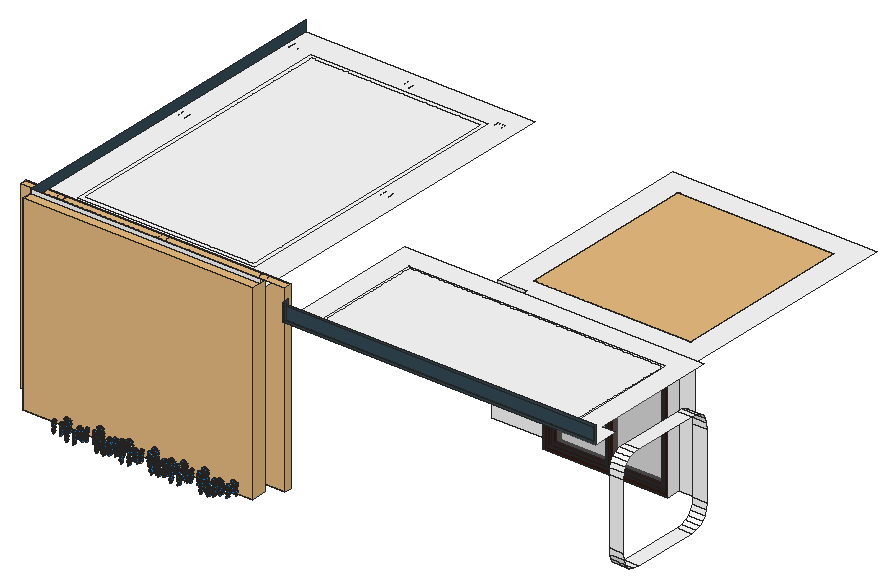
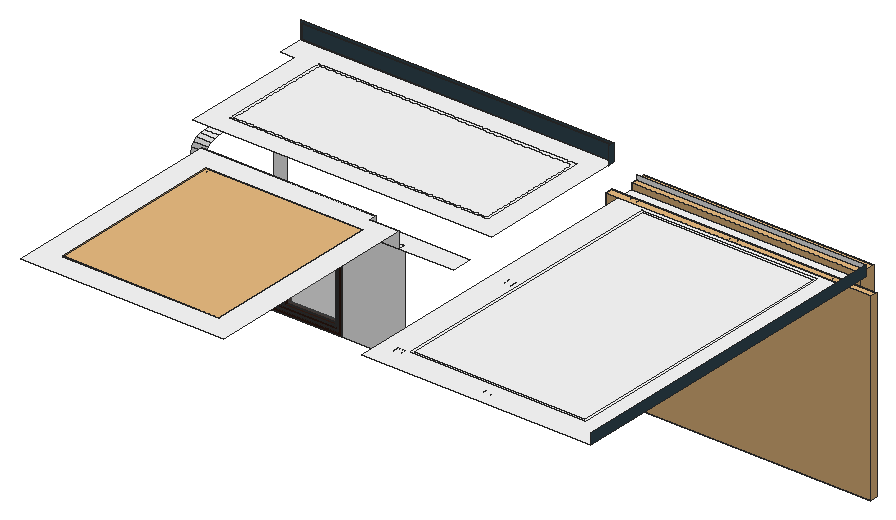
# SketchUp Ruby script. Lengths in inches.
U = 1.inch
M = Sketchup.active_model
def pt(a) = Geom::Point3d.new(a.map { |v| v * U })
def face(e, loops, mat)
  f = e.add_face(loops[0].map { |a| pt(a) })
  loops[1..].each { |l| e.add_face(l.map { |a| pt(a) }).erase! }
  f.material = f.back_material = mat if mat
  f
end
# faces: each face lists its corners as indices into pts; further lists are holes
def faces(e, pts, list, mat = nil) = list.each { |f| face(e, (f[0].is_a?(Array) ? f : [f]).map { |l| l.map { |i| pts[i] } }, mat) }
# xy, xz, yz: faces in a plane at the given z, y or x. An outline is a flat list of corners, or four numbers for a rectangle; further outlines are holes
def ring(l) = l.size == 4 ? [[l[0], l[1]], [l[2], l[1]], [l[2], l[3]], [l[0], l[3]]] : l.each_slice(2).to_a
def flat(e, list, mat, &to3) = list.each { |f| face(e, (f[0].is_a?(Array) ? f : [f]).map { |l| ring(l).map { |u, v| to3.(u, v) } }, mat) }
def xy(e, z, list, mat = nil) = flat(e, list, mat) { |x, y| [x, y, z] }
def xz(e, y, list, mat = nil) = flat(e, list, mat) { |x, z| [x, y, z] }
def yz(e, x, list, mat = nil) = flat(e, list, mat) { |y, z| [x, y, z] }
def lines(e, pts, list) = list.each { |a, b| e.add_line(pt(pts[a]), pt(pts[b])) }
# prism: a flat outline (further loops are holes) pulled along v
def prism(e, loops, v, mat = nil)
  f = face(e, loops, mat); d = Geom::Vector3d.new(v.map { |x| x * U })
  f.pushpull(f.normal.samedirection?(d) ? d.length : -d.length)
end
def box(e, o, s, mat = nil) = prism(e, [[o, [o[0] + s[0], o[1], o[2]], [o[0] + s[0], o[1] + s[1], o[2]], [o[0], o[1] + s[1], o[2]]]], [0, 0, s[2]], mat)
def at(x, y, z, deg = 0) = Geom::Transformation.translation(pt([x, y, z])) * Geom::Transformation.rotation(ORIGIN, Z_AXIS, deg.degrees)
def axes(o, x, y, z) = Geom::Transformation.new([*x, 0, *y, 0, *z, 0, *pt(o).to_a, 1])
def part(name) = M.definitions.add(name)
# library, detail: a bought-in or finely detailed component or shape, given as its bounding box
def library(name, o, s) = part(name).tap { |d| box(d.entities, o, s) }
def detail(e, o, s) = box(e.add_group.entities, o, s)
def put(e, d, t, mat = nil) = e.add_instance(d, t).tap { |i| i.material = mat if mat }
def group(e, t, mat = nil) = e.add_group.tap { |g| g.transformation = t; g.material = mat if mat }.entities
root = M.entities
M.materials.add("0496 AP 9691 Shadow-N").color = [53, 75, 86]
M.materials.add("[Color M00]").color = [255, 255, 255]
M.materials.add("[Translucent Glass Gray]").color = [128, 128, 128]
M.materials["[Translucent Glass Gray]"].alpha = 0.5
M.materials.add("lz-doorbrown").color = [51, 28, 20]
M.materials.add("skp avat flo 1").color = [0, 129, 229]
M.materials.add("skp avat flo 2").color = [47, 120, 22]
c1 = part("Gruppe\#2")
xy(c1.entities,0,[[6.69,0,4.96,0.23,3.03,1.59,1.96,1.96,0.9,3.35,0.9,5.71,0,6.69,0.23,8.43,1.96,10,3.35,12.49,4.67,13.04,7.04,12.49,8.72,13.04,10.04,12.49,11.43,11.43,12.05,9.15,13.39,6.69,13.16,4.96,12.49,3.35,10.41,2.22,8.43,0.23]],"skp avat flo 1")
c2 = part("Gruppe\#12")
xy(c2.entities,0,[[1.18,0.5,1.36,0.52,1.52,0.59,1.67,0.7,1.77,0.84,1.84,1,1.87,1.18,1.84,1.36,1.77,1.52,1.67,1.67,1.52,1.77,1.36,1.84,1.18,1.87,1,1.84,0.84,1.77,0.7,1.67,0.59,1.52,0.52,1.36,0.5,1.18,0.52,1,0.59,0.84,0.7,0.7,0.84,0.59,1,0.52]])
c3 = part("f.st. wop plant 01 blüte")
put(c3.entities,c1,at(0,0,0))
put(c3.entities,c2,at(5.65,5.41,0.39))
c4 = part("Gruppe\#5")
xy(c4.entities,0.96,[[13.97,0.22,8.73,4.42,7.37,10.11,8.43,14.53,13.97,16.39]],"skp avat flo 2")
p = [[13.97,0.22,0.96],[13.97,16.39,0.96],[17.89,14.53,4.875],[18.64,10.11,5.625],[17.67,4.42,4.66]]
faces(c4.entities,p,[[0,1,2,3,4]],"skp avat flo 2")
c5 = part("f.st. wop plant 01 blatt")
put(c5.entities,c4,axes([0.99,0,4.74],[0.91566,0,-0.40195],[0,1,0],[0.40195,0,0.91566]))
c6 = part("Gruppe\#10")
put(c6.entities,c3,axes([4.61,0.45,57.14],[0.99373,-0.06775,-0.08889],[0.11172,0.62588,0.77188],[0.00335,-0.77697,0.62953]))
put(c6.entities,c3,axes([12.4,0.4,0.59],[0.70061,0.70799,-0.08889],[-0.40079,0.49353,0.77188],[0.59035,-0.50516,0.62953]))
put(c6.entities,c3,axes([24.4375,6.09,17.58],[-0.05734,0.99439,-0.08889],[-0.63495,0.03239,0.77188],[0.77043,0.1007,0.62953]))
put(c6.entities,c3,axes([1.11,8.09,13.25],[0.88983,-0.44754,-0.08889],[0.34553,0.53368,0.77188],[-0.298,-0.71756,0.62953]))
put(c6.entities,c3,axes([23.26,15,37.53],[-0.84836,0.52191,-0.08889],[-0.38985,-0.50222,0.77188],[0.35821,0.68948,0.62953]))
put(c6.entities,c3,axes([12.67,23.61,24.88],[-0.75852,-0.64555,-0.08889],[0.35717,-0.52596,0.77188],[-0.54504,0.55374,0.62953]))
put(c6.entities,c3,axes([20.43,22.9,81.42],[-0.98432,0.15238,-0.08889],[-0.16477,-0.61405,0.77188],[0.06303,0.77442,0.62953]))
put(c6.entities,c3,axes([1.76,2.9,29.21],[0.93833,-0.33412,-0.08889],[0.27691,0.5723,0.77188],[-0.20703,-0.74889,0.62953]))
put(c6.entities,c3,axes([13.59,0.5,77.09],[0.62412,0.77625,-0.08889],[-0.4494,0.44972,0.77188],[0.63915,-0.4418,0.62953]))
put(c6.entities,c3,axes([-1.26,15.51,69.79],[0.24265,-0.96603,-0.08889],[0.62977,0.08716,0.77188],[-0.73791,-0.24328,0.62953]))
put(c6.entities,c3,axes([22.04,17.92,65.46],[-0.95793,0.27287,-0.08889],[-0.2394,-0.58898,0.77188],[0.15827,0.76069,0.62953]))
put(c6.entities,c3,axes([9.51,23.35,52.81],[-0.55554,-0.82673,-0.08889],[0.48617,-0.40969,0.77188],[-0.67455,0.38559,0.62953]))
put(c6.entities,c3,axes([0.1875,18.97,41.86],[-0.02781,-0.99565,-0.08889],[0.62986,-0.08651,0.77188],[-0.77621,-0.03452,0.62953]))
put(c6.entities,c3,axes([24.98,7.4,94.08],[-0.15925,0.98323,-0.08889],[-0.63491,-0.03305,0.77188],[0.75599,0.17936,0.62953]))
put(c6.entities,c3,axes([21.5,21.98,4.93],[-0.96344,0.25275,-0.08889],[-0.22702,-0.59386,0.77188],[0.1423,0.76384,0.62953]))
put(c6.entities,c3,axes([1.57,6.98,89.75],[0.93112,-0.3537,-0.08889],[0.28884,0.56637,0.77188],[-0.22267,-0.74439,0.62953]))
put(c6.entities,c5,axes([9.37,32.32,90.95],[-0.51317,-0.65235,0],[0.5996,-0.47167,0.32697],[-0.25699,0.20216,0.76288]))
put(c6.entities,c5,axes([33.81,6.72,78.35],[-0.27992,0.78137,0],[-0.71819,-0.25729,0.32697],[0.30782,0.11027,0.76288]))
put(c6.entities,c5,axes([-9.46,14.86,61.47],[0.53029,-0.63851,0],[0.58688,0.4874,0.32697],[-0.25154,-0.2089,0.76288]))
put(c6.entities,c5,axes([21.49,-6.15,66.98],[0.2591,0.78852,0],[-0.72476,0.23815,0.32697],[0.31063,-0.10207,0.76288]))
put(c6.entities,c5,axes([32.03,5.27,54.38],[-0.36397,0.74594,0],[-0.68562,-0.33454,0.32697],[0.29386,0.14338,0.76288]))
put(c6.entities,c5,axes([30.63,20.6,49.31],[-0.77544,0.29596,0],[-0.27203,-0.71273,0.32697],[0.11659,0.30548,0.76288]))
put(c6.entities,c5,axes([32.03,5.27,27.16],[-0.36397,0.74594,0],[-0.68562,-0.33454,0.32697],[0.29386,0.14338,0.76288]))
put(c6.entities,c5,axes([17.4375,27.53,13.8125],[-0.76735,-0.23527,0.21148],[0.29408,-0.735,0.24937],[0.11659,0.30548,0.76288]))
put(c6.entities,c5,axes([-9.46,14.86,34.24],[0.53029,-0.63851,0],[0.58688,0.4874,0.32697],[-0.25154,-0.2089,0.76288]))
c7 = part("Gruppe\#9")
put(c7.entities,c3,axes([2.2,1.62,57.61],[0.97169,-0.0623,-0.22792],[0.22172,0.57378,0.78843],[0.08166,-0.81664,0.57134]))
put(c7.entities,c3,axes([-1.48,7.53,1.27],[0.68093,0.71536,-0.15682],[-0.22028,0.40428,0.88771],[0.69843,-0.56993,0.43287]))
put(c7.entities,c3,axes([13.97,11.34,15.86],[-0.0542,0.99797,0.03349],[-0.45869,-0.05467,0.88691],[0.88694,0.03271,0.46072]))
put(c7.entities,c3,axes([-9.71,13.74,16.77],[0.84218,-0.4326,-0.32186],[0.5102,0.4462,0.73526],[-0.17446,-0.78343,0.59649]))
put(c7.entities,c3,axes([17.17,17.99,36.46],[-0.83727,0.52624,0.14846],[-0.23006,-0.58536,0.77745],[0.49603,0.61679,0.61117]))
put(c7.entities,c3,axes([4.35,27.92,27.32],[-0.77345,-0.63385,0.00301],[0.4998,-0.60694,0.61792],[-0.38984,0.47943,0.78623]))
put(c7.entities,c3,axes([20.43,22.9,81.42],[-0.98432,0.15238,-0.08889],[-0.16477,-0.61405,0.77188],[0.06303,0.77442,0.62953]))
put(c7.entities,c3,axes([-5.84,6.82,31.58],[0.89192,-0.31974,-0.31975],[0.44391,0.4844,0.75386],[-0.08616,-0.81432,0.57398]))
put(c7.entities,c3,axes([13.59,0.5,77.09],[0.62412,0.77625,-0.08889],[-0.4494,0.44972,0.77188],[0.63915,-0.4418,0.62953]))
put(c7.entities,c3,axes([-1.26,15.51,69.79],[0.24265,-0.96603,-0.08889],[0.62977,0.08716,0.77188],[-0.73791,-0.24328,0.62953]))
put(c7.entities,c3,axes([20.77,18.5,64.59],[-0.95848,0.27864,0.06062],[-0.13765,-0.63827,0.75741],[0.24973,0.71762,0.65012]))
put(c7.entities,c3,axes([6.6875,24.75,54.15],[-0.57029,-0.8188,-0.06577],[0.58283,-0.45976,0.67002],[-0.57885,0.34377,0.73942]))
put(c7.entities,c3,axes([-4.08,21.11,44.3125],[-0.04911,-0.98765,-0.14878],[0.72825,-0.13735,0.67141],[-0.68355,-0.07538,0.726]))
put(c7.entities,c3,axes([24.98,7.4,94.08],[-0.15925,0.98323,-0.08889],[-0.63491,-0.03305,0.77188],[0.75599,0.17936,0.62953]))
put(c7.entities,c3,axes([8.77,28.52,5.9],[-0.95532,0.25842,0.14346],[-0.07274,-0.676,0.7333],[0.28648,0.6901,0.6646]))
put(c7.entities,c3,axes([1.57,6.98,89.75],[0.93112,-0.3537,-0.08889],[0.28884,0.56637,0.77188],[-0.22267,-0.74439,0.62953]))
put(c7.entities,c5,axes([9.37,32.32,90.95],[-0.51317,-0.65235,0],[0.5996,-0.47167,0.32697],[-0.25699,0.20216,0.76288]))
put(c7.entities,c5,axes([33.81,6.72,78.35],[-0.27992,0.78137,0],[-0.71819,-0.25729,0.32697],[0.30782,0.11027,0.76288]))
put(c7.entities,c5,axes([-11.01,15.72,64.74],[0.51926,-0.63742,-0.11388],[0.63054,0.46456,0.27478],[-0.14729,-0.25842,0.77487]))
put(c7.entities,c5,axes([20.21,-5.625,64.6],[0.26417,0.78668,0.01588],[-0.67119,0.21655,0.43762],[0.41063,-0.15212,0.70508]))
put(c7.entities,c5,axes([29.04,6.59,51.45],[-0.35348,0.74452,0.09816],[-0.63785,-0.35493,0.39506],[0.39635,0.09281,0.72332]))
put(c7.entities,c5,axes([27.11,22.23,47.625],[-0.76537,0.29574,0.12508],[-0.23173,-0.73252,0.31403],[0.22228,0.25465,0.75805]))
put(c7.entities,c5,axes([23.375,9.49,23.48],[-0.34051,0.7404,0.15735],[-0.60881,-0.37042,0.42548],[0.44978,0.05914,0.69506]))
put(c7.entities,c5,axes([6.77,33.04,15.99],[-0.71083,-0.25923,0.3412],[0.32455,-0.75723,0.10082],[0.2798,0.21977,0.74988]))
put(c7.entities,c5,axes([-15.51,18.125,40.12],[0.50532,-0.63318,-0.18065],[0.65217,0.44994,0.24724],[-0.09068,-0.29247,0.77145]))
c8 = part("Gruppe\#11")
put(c8.entities,c3,axes([4.61,0.45,57.14],[0.99373,-0.06775,-0.08889],[0.11172,0.62588,0.77188],[0.00335,-0.77697,0.62953]))
put(c8.entities,c3,axes([12.4,0.4,0.59],[0.70061,0.70799,-0.08889],[-0.40079,0.49353,0.77188],[0.59035,-0.50516,0.62953]))
put(c8.entities,c3,axes([24.4375,6.09,17.58],[-0.05734,0.99439,-0.08889],[-0.63495,0.03239,0.77188],[0.77043,0.1007,0.62953]))
put(c8.entities,c3,axes([1.11,8.09,13.25],[0.88983,-0.44754,-0.08889],[0.34553,0.53368,0.77188],[-0.298,-0.71756,0.62953]))
put(c8.entities,c3,axes([23.26,15,37.53],[-0.84836,0.52191,-0.08889],[-0.38985,-0.50222,0.77188],[0.35821,0.68948,0.62953]))
put(c8.entities,c3,axes([12.67,23.61,24.88],[-0.75852,-0.64555,-0.08889],[0.35717,-0.52596,0.77188],[-0.54504,0.55374,0.62953]))
put(c8.entities,c3,axes([20.43,22.9,81.42],[-0.98432,0.15238,-0.08889],[-0.16477,-0.61405,0.77188],[0.06303,0.77442,0.62953]))
put(c8.entities,c3,axes([1.76,2.9,29.21],[0.93833,-0.33412,-0.08889],[0.27691,0.5723,0.77188],[-0.20703,-0.74889,0.62953]))
put(c8.entities,c3,axes([13.59,0.5,77.09],[0.62412,0.77625,-0.08889],[-0.4494,0.44972,0.77188],[0.63915,-0.4418,0.62953]))
put(c8.entities,c3,axes([-1.26,15.51,69.79],[0.24265,-0.96603,-0.08889],[0.62977,0.08716,0.77188],[-0.73791,-0.24328,0.62953]))
put(c8.entities,c3,axes([22.04,17.92,65.46],[-0.95793,0.27287,-0.08889],[-0.2394,-0.58898,0.77188],[0.15827,0.76069,0.62953]))
put(c8.entities,c3,axes([9.51,23.35,52.81],[-0.55554,-0.82673,-0.08889],[0.48617,-0.40969,0.77188],[-0.67455,0.38559,0.62953]))
put(c8.entities,c3,axes([0.1875,18.97,41.86],[-0.02781,-0.99565,-0.08889],[0.62986,-0.08651,0.77188],[-0.77621,-0.03452,0.62953]))
put(c8.entities,c3,axes([24.98,7.4,94.08],[-0.15925,0.98323,-0.08889],[-0.63491,-0.03305,0.77188],[0.75599,0.17936,0.62953]))
put(c8.entities,c3,axes([21.5,21.98,4.93],[-0.96344,0.25275,-0.08889],[-0.22702,-0.59386,0.77188],[0.1423,0.76384,0.62953]))
put(c8.entities,c3,axes([1.57,6.98,89.75],[0.93112,-0.3537,-0.08889],[0.28884,0.56637,0.77188],[-0.22267,-0.74439,0.62953]))
put(c8.entities,c5,axes([9.37,32.32,90.95],[-0.51317,-0.65235,0],[0.5996,-0.47167,0.32697],[-0.25699,0.20216,0.76288]))
put(c8.entities,c5,axes([33.81,6.72,78.35],[-0.27992,0.78137,0],[-0.71819,-0.25729,0.32697],[0.30782,0.11027,0.76288]))
put(c8.entities,c5,axes([-9.46,14.86,61.47],[0.53029,-0.63851,0],[0.58688,0.4874,0.32697],[-0.25154,-0.2089,0.76288]))
put(c8.entities,c5,axes([21.49,-6.15,66.98],[0.2591,0.78852,0],[-0.72476,0.23815,0.32697],[0.31063,-0.10207,0.76288]))
put(c8.entities,c5,axes([32.03,5.27,54.38],[-0.36397,0.74594,0],[-0.68562,-0.33454,0.32697],[0.29386,0.14338,0.76288]))
put(c8.entities,c5,axes([30.63,20.6,49.31],[-0.77544,0.29596,0],[-0.27203,-0.71273,0.32697],[0.11659,0.30548,0.76288]))
put(c8.entities,c5,axes([32.03,5.27,27.16],[-0.36397,0.74594,0],[-0.68562,-0.33454,0.32697],[0.29386,0.14338,0.76288]))
put(c8.entities,c5,axes([17.4375,27.53,13.8125],[-0.76735,-0.23527,0.21148],[0.29408,-0.735,0.24937],[0.11659,0.30548,0.76288]))
put(c8.entities,c5,axes([-9.46,14.86,34.24],[0.53029,-0.63851,0],[0.58688,0.4874,0.32697],[-0.25154,-0.2089,0.76288]))
c9 = part("Gruppe\#8")
put(c9.entities,c3,axes([2.26,1.13,59.39],[0.92531,-0.05375,-0.37538],[0.3384,0.56379,0.75341],[0.17114,-0.82417,0.53987]))
put(c9.entities,c3,axes([-9.39,6.25,4.33],[0.64151,0.72107,-0.26176],[-0.09814,0.41557,0.90425],[0.76081,-0.5544,0.33735]))
put(c9.entities,c3,axes([7.9,10.48,16.53],[-0.06325,0.99763,0.02691],[-0.32763,-0.04623,0.94367],[0.94269,0.05087,0.32978]))
put(c9.entities,c3,axes([-15.4375,12.6,20.76],[0.79424,-0.42729,-0.43198],[0.60271,0.46401,0.64918],[-0.07695,-0.77596,0.62607]))
put(c9.entities,c3,axes([13.9,17.49,36.37],[-0.81529,0.51823,0.25834],[-0.1092,-0.57574,0.81031],[0.56867,0.63242,0.52599]))
put(c9.entities,c3,axes([-0.23,27.12,29.01],[-0.75604,-0.64315,0.1215],[0.59094,-0.59091,0.5492],[-0.28142,0.48702,0.82681]))
put(c9.entities,c3,axes([20.43,22.9,81.42],[-0.98432,0.15238,-0.08889],[-0.16477,-0.61405,0.77188],[0.06303,0.77442,0.62953]))
put(c9.entities,c3,axes([-9.41,5.97,34.96],[0.84215,-0.31382,-0.43852],[0.53918,0.50168,0.67646],[0.00771,-0.80612,0.5917]))
put(c9.entities,c3,axes([13.59,0.5,77.09],[0.62412,0.77625,-0.08889],[-0.4494,0.44972,0.77188],[0.63915,-0.4418,0.62953]))
put(c9.entities,c3,axes([-1.26,15.51,69.79],[0.24265,-0.96603,-0.08889],[0.62977,0.08716,0.77188],[-0.73791,-0.24328,0.62953]))
put(c9.entities,c3,axes([22.04,17.92,65.46],[-0.95793,0.27287,-0.08889],[-0.2394,-0.58898,0.77188],[0.15827,0.76069,0.62953]))
put(c9.entities,c3,axes([6.08,24.33,55.62],[-0.57097,-0.82091,0.01051],[0.68037,-0.46598,0.56565],[-0.45945,0.33012,0.82458]))
put(c9.entities,c3,axes([-6.06,20.77,47.51],[-0.06819,-0.9857,-0.15407],[0.82323,-0.14283,0.54945],[-0.56361,-0.08937,0.8212]))
put(c9.entities,c3,axes([24.98,7.4,94.08],[-0.15925,0.98323,-0.08889],[-0.63491,-0.03305,0.77188],[0.75599,0.17936,0.62953]))
put(c9.entities,c3,axes([1.11,27.4375,7.17],[-0.92899,0.24893,0.27387],[0.04156,-0.66514,0.74556],[0.36776,0.70401,0.60756]))
put(c9.entities,c3,axes([1.57,6.98,89.75],[0.93112,-0.3537,-0.08889],[0.28884,0.56637,0.77188],[-0.22267,-0.74439,0.62953]))
put(c9.entities,c5,axes([9.37,32.32,90.95],[-0.51317,-0.65235,0],[0.5996,-0.47167,0.32697],[-0.25699,0.20216,0.76288]))
put(c9.entities,c5,axes([33.81,6.72,78.35],[-0.27992,0.78137,0],[-0.71819,-0.25729,0.32697],[0.30782,0.11027,0.76288]))
put(c9.entities,c5,axes([-9.74,15.05,68.68],[0.49765,-0.63289,-0.20172],[0.66377,0.46408,0.1815],[-0.02561,-0.27014,0.78439]))
put(c9.entities,c5,axes([21.49,-6.15,66.98],[0.2591,0.78852,0],[-0.72476,0.23815,0.32697],[0.31063,-0.10207,0.76288]))
put(c9.entities,c5,axes([27.8125,6.34,49.26],[-0.33661,0.74111,0.1623],[-0.5684,-0.36396,0.48306],[0.5025,0.08476,0.65514]))
put(c9.entities,c5,axes([25.26,22.01,46],[-0.73801,0.28975,0.24554],[-0.17833,-0.73814,0.33502],[0.33532,0.24514,0.71859]))
put(c9.entities,c5,axes([18.32,8.86,22.77],[-0.32541,0.73857,0.19371],[-0.53703,-0.37106,0.51265],[0.54278,0.07565,0.62335]))
put(c9.entities,c5,axes([0.49,32.09,17.38],[-0.65154,-0.26248,0.44214],[0.34641,-0.75151,0.06433],[0.37999,0.23503,0.69948]))
put(c9.entities,c5,axes([-17.94,17.29,44.63],[0.48369,-0.62973,-0.24163],[0.67408,0.46176,0.14595],[0.0237,-0.2813,0.78052]))
c10 = part("f.st. wop plant 01")
put(c10.entities,c6,at(39.14,64.09,18.66,-141.2))
put(c10.entities,c7,axes([53.54,120.93,12.24],[-0.61849,0.75929,0.20233],[-0.78178,-0.62056,-0.06099],[0.07925,-0.1959,0.97742]))
put(c10.entities,c8,at(82.26,36.89,18.66))
put(c10.entities,c9,axes([72.55,-5.87,29.3],[0.62579,-0.70508,0.33355],[0.76326,0.64164,-0.07566],[-0.16067,0.30193,0.93969]))
c11 = part("World of Pandora - tree 01")
put(c11.entities,c10,at(57.06,8.63,0))
c12 = library("Sliding windows",[335.6875,-0.89,0.35],[144.14,8.85,122.84])
c13 = library("шторы раздвинутые\#1",[23.6875,-79.1875,2.97],[68.3125,79.67,3.21])
c14 = part("window full")
xy(c14.entities,0,[[0,0,14.17,66.54]],"lz-doorbrown")
xy(c14.entities,2.26,[[12.2,2.26,14.17,64.28]],"lz-doorbrown")
xy(c14.entities,2.36,[[0,2.36,1.97,64.17]],"lz-doorbrown")
xy(c14.entities,3.74,[[11.42,3.74,12.2,32.875],[11.42,33.66,12.2,62.79]],"lz-doorbrown")
xy(c14.entities,3.9375,[[1.97,3.9375,2.76,32.77],[1.97,33.76,2.76,62.6]],"lz-doorbrown")
xy(c14.entities,4.18,[[2.76,4.18,7.09,32.09],[7.09,4.18,11.42,32.09],[2.76,34.45,7.09,62.35],[7.09,34.45,11.42,62.35]],"lz-doorbrown")
xy(c14.entities,69.83,[[2.76,4.18,7.09,32.09],[7.09,4.18,11.42,32.09],[7.09,32.09,11.42,34.45],[2.76,34.45,7.09,62.35],[7.09,34.45,11.42,62.35]],"lz-doorbrown")
xy(c14.entities,70.08,[[1.97,3.9375,2.76,32.77],[1.97,33.76,2.76,62.6]],"lz-doorbrown")
xy(c14.entities,70.27,[[11.42,3.74,12.2,32.875],[11.42,32.875,12.2,33.66],[11.42,33.66,12.2,62.79]],"lz-doorbrown")
xy(c14.entities,71.65,[[0,2.36,1.97,64.17]],"lz-doorbrown")
xy(c14.entities,71.76,[[12.2,2.26,14.17,64.28]],"lz-doorbrown")
xy(c14.entities,74.02,[[0,0,14.17,66.54]],"lz-doorbrown")
xz(c14.entities,0,[[0,0,14.17,74.02]],"lz-doorbrown")
xz(c14.entities,2.26,[[12.2,2.26,14.17,71.76]],"lz-doorbrown")
xz(c14.entities,2.36,[[0,2.36,1.97,71.65]],"lz-doorbrown")
xz(c14.entities,3.74,[[11.42,3.74,12.2,70.27]],"lz-doorbrown")
xz(c14.entities,3.9375,[[1.97,3.9375,2.76,70.08]],"lz-doorbrown")
xz(c14.entities,4.18,[[2.76,4.18,7.09,69.83],[7.09,4.18,11.42,69.83]],"lz-doorbrown")
xz(c14.entities,32.09,[[2.76,4.18,11.42,69.83]],"lz-doorbrown")
xz(c14.entities,32.77,[[1.97,3.9375,2.76,70.08]],"lz-doorbrown")
xz(c14.entities,32.875,[[11.42,3.74,12.2,70.27]],"lz-doorbrown")
xz(c14.entities,33.66,[[11.42,3.74,12.2,47.88],[11.42,47.88,12.2,70.27]],"lz-doorbrown")
xz(c14.entities,33.76,[[1.97,3.9375,2.76,70.08]],"lz-doorbrown")
xz(c14.entities,34.45,[[2.76,4.18,11.42,69.83]],"lz-doorbrown")
xz(c14.entities,62.35,[[2.76,4.18,7.09,69.83],[7.09,4.18,11.42,69.83]],"lz-doorbrown")
xz(c14.entities,62.6,[[1.97,3.9375,2.76,70.08]],"lz-doorbrown")
xz(c14.entities,62.79,[[11.42,3.74,12.2,70.27]],"lz-doorbrown")
xz(c14.entities,64.17,[[0,2.36,1.97,71.65]],"lz-doorbrown")
xz(c14.entities,64.28,[[12.2,2.26,14.17,71.76]],"lz-doorbrown")
xz(c14.entities,66.54,[[0,0,14.17,74.02]],"lz-doorbrown")
yz(c14.entities,0,[[[0,0,66.54,74.02],[2.36,2.36,64.17,71.65]]],"lz-doorbrown")
yz(c14.entities,1.97,[[[2.36,2.36,64.17,71.65],[33.76,3.9375,62.6,70.08],[3.9375,3.9375,32.77,70.08]]],"lz-doorbrown")
yz(c14.entities,2.76,[[[3.9375,3.9375,32.77,70.08],[4.18,4.18,32.09,69.83]],[32.77,3.9375,33.76,4.18],[[33.76,3.9375,62.6,70.08],[34.45,4.18,62.35,69.83]],[32.77,4.18,33.76,69.83],[32.77,69.83,33.76,70.08]],"lz-doorbrown")
yz(c14.entities,7.09,[[4.18,4.18,62.35,69.83]],"[Translucent Glass Gray]")
yz(c14.entities,11.42,[[[3.74,3.74,32.875,70.27],[4.18,4.18,32.09,69.83]],[[33.66,3.74,62.79,70.27],[34.45,4.18,62.35,69.83]],[32.875,69.83,33.66,70.27]],"lz-doorbrown")
yz(c14.entities,12.2,[[[2.26,2.26,64.28,71.76],[3.74,3.74,32.875,70.27],[33.66,3.74,62.79,70.27]]],"lz-doorbrown")
yz(c14.entities,14.17,[[[0,0,66.54,74.02],[2.26,2.26,64.28,71.76]]],"lz-doorbrown")
p = [[11.42,32.875,70.27],[11.42,32.875,70.28]]
lines(c14.entities,p,[[0,1]])
c15 = library("Group\#197",[-0.5,-0.5,-0.1],[90,103.375,0.2])
c16 = part("Group\#6")
xy(c16.entities,0,[[1.28,0,0.95,0.04,0.64,0.17,0.375,0.375,0.17,0.64,0.04,0.95,0,1.28,0.04,1.61,0.17,1.92,0.375,2.18,0.64,2.39,0.95,2.51,1.28,2.56,1.61,2.51,1.92,2.39,2.18,2.18,2.39,1.92,2.51,1.61,2.56,1.28,2.51,0.95,2.39,0.64,2.18,0.375,1.92,0.17,1.61,0.04]])
c17 = part("Group\#12")
detail(c17.entities,[2.45,2.45,12.38],[4,4,0.32])
put(c17.entities,c16,at(3.17,3.17,12.51),"[Color M00]")
xy(root,49,[[1316.11,234.26,1324.11,272.24],[1223.61,291.25,1295.36,299.25]],"[Color M00]")
xy(root,109,[[1316.11,234.26,1324.11,272.24],[1156.42,291.25,1156.42,303.3125,1187.61,303.3125,1187.61,299.25,1204.42,299.25,1204.42,291.25],[1223.61,291.25,1295.36,299.25],[1187.61,299.25,1204.42,303.3125]],"[Color M00]")
xy(root,118.25,[[[1204.42,299.25,1204.42,303.3125,1187.61,303.3125,1187.61,429.625,1304.61,429.625,1304.61,299.25],[1218.42,313.25,1290.61,313.25,1290.61,415.625,1201.61,415.625,1201.61,317.3125,1218.42,317.3125]],[1220.42,315.25,1220.42,319.3125,1203.61,319.3125,1203.61,413.625,1288.61,413.625,1288.61,315.25]],"[Color M00]")
xy(root,125,[[[1144.11,203.25,1144.11,291.25,1316.11,291.25,1316.11,217.8125,1324.11,217.8125,1324.11,203.25],[1156.11,215.25,1304.11,279.25]],[1157.41,216.55,1302.8125,277.95]],"[Color M00]")
xy(root,126,[[1145.11,203.25,1323.11,204.25]],"0496 AP 9691 Shadow-N")
xy(root,127,[[[988.11,217.0625,1120.11,414.75],[1003.11,232.0625,1105.11,399.75]],[1005.11,234.0625,1103.11,397.75]],"[Color M00]")
xz(root,203.25,[[[1144.11,125,1324.11,135],[1145.11,126,1323.11,134]]],"0496 AP 9691 Shadow-N")
xz(root,204.25,[[1145.11,126,1323.11,134]],"0496 AP 9691 Shadow-N")
xz(root,217.0625,[[988.11,127,1120.11,133]],"[Color M00]")
xz(root,223.25,[[1316.11,60.01,1324.11,97.99]],"[Color M00]")
xz(root,283.25,[[1316.11,60.01,1324.11,97.99]],"[Color M00]")
xz(root,299.25,[[1187.61,49,1187.61,109,1204.42,109,1204.42,118.25,1223.61,118.25,1223.61,49],[1295.36,49,1304.61,118.25],[1223.61,109,1295.36,118.25]],"[Color M00]")
xz(root,303.3125,[[1187.61,109,1204.42,118.25]],"[Color M00]")
yz(root,988.11,[[217.0625,127,414.75,133]],"0496 AP 9691 Shadow-N")
yz(root,1144.11,[[203.25,125,207.25,135]],"0496 AP 9691 Shadow-N")
yz(root,1145.11,[[203.25,126,204.25,134]],"0496 AP 9691 Shadow-N")
yz(root,1204.42,[[299.25,109,303.3125,118.25]],"[Color M00]")
yz(root,1223.61,[[291.25,49,299.25,109]],"[Color M00]")
yz(root,1295.36,[[291.25,49,299.25,109]],"[Color M00]")
yz(root,1323.11,[[203.25,126,204.25,134]],"0496 AP 9691 Shadow-N")
p = [[1316.11,230.89,49.31],[1324.11,230.89,49.31],[1324.11,234.26,49],[1316.11,234.26,49],[1316.11,272.24,49],[1324.11,272.24,49],
  [1324.11,275.61,49.31],[1316.11,275.61,49.31],[1316.11,228.14,50.22],[1324.11,228.14,50.22],[1324.11,278.36,50.22],[1316.11,278.36,50.22],
  [1316.11,226,51.75],[1324.11,226,51.75],[1324.11,280.5,51.75],[1316.11,280.5,51.75],[1316.11,224.47,53.89],[1324.11,224.47,53.89],
  [1324.11,282.03,53.89],[1316.11,282.03,53.89],[1316.11,223.56,56.64],[1324.11,223.56,56.64],[1324.11,282.94,56.64],[1316.11,282.94,56.64],
  [1316.11,223.25,60.01],[1324.11,223.25,60.01],[1324.11,283.25,60.01],[1316.11,283.25,60.01],[1316.11,223.56,101.36],[1324.11,223.56,101.36],
  [1324.11,223.25,97.99],[1316.11,223.25,97.99],[1324.11,282.94,101.36],[1316.11,282.94,101.36],[1316.11,283.25,97.99],[1324.11,283.25,97.99],
  [1316.11,224.47,104.11],[1324.11,224.47,104.11],[1324.11,282.03,104.11],[1316.11,282.03,104.11],[1316.11,226,106.25],[1324.11,226,106.25],
  [1324.11,280.5,106.25],[1316.11,280.5,106.25],[1316.11,228.14,107.78],[1324.11,228.14,107.78],[1324.11,278.36,107.78],[1316.11,278.36,107.78],
  [1316.11,230.89,108.69],[1324.11,230.89,108.69],[1324.11,275.61,108.69],[1316.11,275.61,108.69],[1316.11,234.26,109],[1324.11,234.26,109],
  [1324.11,272.24,109],[1316.11,272.24,109]]
faces(root,p,[[0,1,2,3],[4,5,6,7],[8,9,1,0],[7,6,10,11],[12,13,9,8],[11,10,14,15],[16,17,13,12],[15,14,18,19],
  [20,21,17,16],[19,18,22,23],[24,25,21,20],[23,22,26,27],[28,29,30,31],[32,33,34,35],[36,37,29,28],[38,39,33,32],
  [40,41,37,36],[42,43,39,38],[44,45,41,40],[46,47,43,42],[48,49,45,44],[50,51,47,46],[52,53,49,48],[54,55,51,50]],"[Color M00]")
put(root,c11,axes([1045,197.47,18.55],[-0.00253,0.07025,0],[-0.07025,-0.00253,0],[0,0,0.0703]))
put(root,c11,axes([1076.4375,197.47,18.55],[-0.00253,0.07025,0],[-0.07025,-0.00253,0],[0,0,0.0703]))
put(root,c11,axes([1105.125,197.47,18.55],[-0.00253,0.07025,0],[-0.07025,-0.00253,0],[0,0,0.0703]))
put(root,c11,axes([1028.24,196.87,18.62],[-0.00253,0.07025,0],[-0.07025,-0.00253,0],[0,0,0.0703]))
put(root,c11,axes([1059.67,196.87,18.62],[-0.00253,0.07025,0],[-0.07025,-0.00253,0],[0,0,0.0703]))
put(root,c11,axes([1088.36,196.87,18.62],[-0.00253,0.07025,0],[-0.07025,-0.00253,0],[0,0,0.0703]))
put(root,c11,axes([1048.26,197.32,19.63],[-0.00253,0.07025,0],[-0.07025,-0.00253,0],[0,0,0.0703]))
put(root,c11,axes([1079.7,197.32,19.63],[-0.00253,0.07025,0],[-0.07025,-0.00253,0],[0,0,0.0703]))
put(root,c11,axes([1108.38,197.32,19.63],[-0.00253,0.07025,0],[-0.07025,-0.00253,0],[0,0,0.0703]))
put(root,c11,axes([1058.2,221.5,19.95],[-0.07025,-0.00253,0],[0.00253,-0.07025,0],[0,0,0.0703]))
put(root,c11,axes([1089.64,221.5,19.95],[-0.07025,-0.00253,0],[0.00253,-0.07025,0],[0,0,0.0703]))
put(root,c11,axes([1118.32,221.5,19.95],[-0.07025,-0.00253,0],[0.00253,-0.07025,0],[0,0,0.0703]))
put(root,c11,axes([1020.51,197.22,20.27],[-0.00253,0.07025,0],[-0.07025,-0.00253,0],[0,0,0.0703]))
put(root,c11,axes([1051.95,197.22,20.27],[-0.00253,0.07025,0],[-0.07025,-0.00253,0],[0,0,0.0703]))
put(root,c11,axes([1080.63,197.22,20.27],[-0.00253,0.07025,0],[-0.07025,-0.00253,0],[0,0,0.0703]))
put(root,c11,axes([1054.99,198.59,20.74],[-0.00253,0.07025,0],[-0.07025,-0.00253,0],[0,0,0.0703]))
put(root,c11,axes([1086.43,198.59,20.74],[-0.00253,0.07025,0],[-0.07025,-0.00253,0],[0,0,0.0703]))
put(root,c11,axes([1115.12,198.59,20.74],[-0.00253,0.07025,0],[-0.07025,-0.00253,0],[0,0,0.0703]))
put(root,c12,axes([680.7,212.47,21.1875],[0.91577,0,0],[0,1,0],[0,0,0.88737]))
put(root,c11,axes([1037.76,199.29,21.04],[-0.00253,0.07025,0],[-0.07025,-0.00253,0],[0,0,0.0703]))
put(root,c11,axes([1069.19,199.29,21.04],[-0.00253,0.07025,0],[-0.07025,-0.00253,0],[0,0,0.0703]))
put(root,c11,axes([1097.88,199.29,21.04],[-0.00253,0.07025,0],[-0.07025,-0.00253,0],[0,0,0.0703]))
put(root,c13,axes([922.04,233.22,126.375],[2.23186,0,0],[0,0,1.3214],[0,-1.17,0]))
put(root,c14,axes([1223.89,299.0625,49.05],[0,-0.54,0],[1.07,0,0],[0,0,0.81]))
put(root,c15,at(1201.61,313.25,118.25),"0496 AP 9691 Shadow-N")
g1 = group(root,at(1156.11,215.25,125),"0496 AP 9691 Shadow-N")
xy(g1,0,[[[0,0,148,64],[1.3,1.3,146.7,62.7]]],"[Color M00]")
put(root,c17,at(992.24,223.62,113.99),"0496 AP 9691 Shadow-N")
put(root,c17,at(1051.24,223.62,113.99),"0496 AP 9691 Shadow-N")
put(root,c17,at(1108.99,223.62,113.99),"0496 AP 9691 Shadow-N")
put(root,c17,at(1105.08,316.86,113.99),"0496 AP 9691 Shadow-N")
put(root,c17,at(988.33,316.86,113.99),"0496 AP 9691 Shadow-N")
put(root,c17,at(988.33,397.05,113.99),"0496 AP 9691 Shadow-N")
put(root,c17,at(1105.08,397.05,113.99),"0496 AP 9691 Shadow-N")
put(root,c17,at(1049.87,401.37,113.99),"0496 AP 9691 Shadow-N")
g2 = group(root,at(1003.11,232.0625,127),"0496 AP 9691 Shadow-N")
xy(g2,0,[[[0,0,102,167.6875],[2,2,100,165.6875]]],"[Color M00]")
